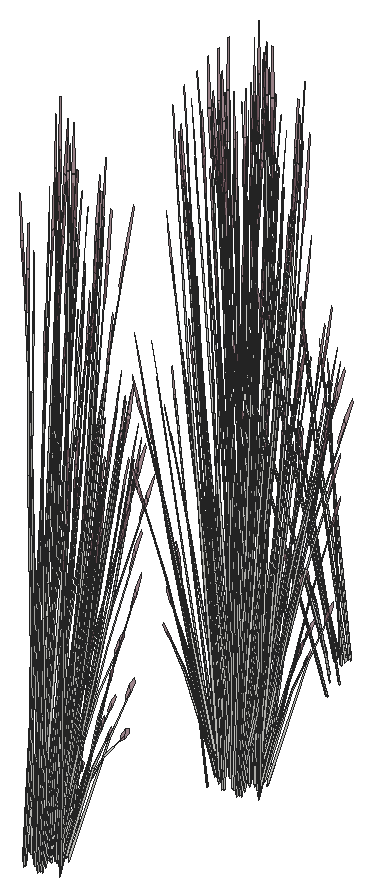
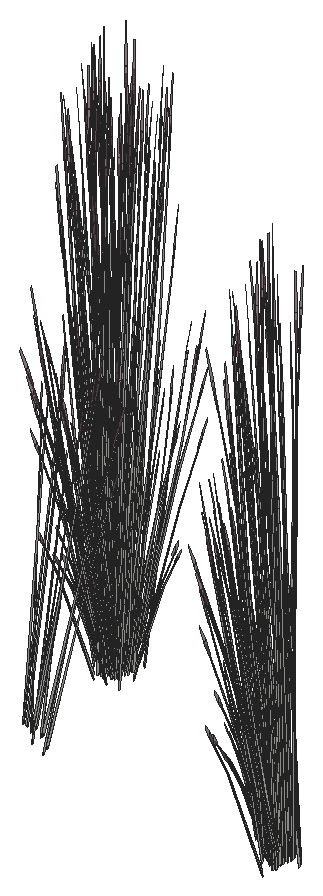
# SketchUp Ruby script. Lengths in inches.
U = 1.inch
M = Sketchup.active_model
def pt(a) = Geom::Point3d.new(a.map { |v| v * U })
def face(e, loops, mat)
  f = e.add_face(loops[0].map { |a| pt(a) })
  loops[1..].each { |l| e.add_face(l.map { |a| pt(a) }).erase! }
  f.material = f.back_material = mat if mat
  f
end
# faces: each face lists its corners as indices into pts; further lists are holes
def faces(e, pts, list, mat = nil) = list.each { |f| face(e, (f[0].is_a?(Array) ? f : [f]).map { |l| l.map { |i| pts[i] } }, mat) }
# xy, xz, yz: faces in a plane at the given z, y or x. An outline is a flat list of corners, or four numbers for a rectangle; further outlines are holes
def ring(l) = l.size == 4 ? [[l[0], l[1]], [l[2], l[1]], [l[2], l[3]], [l[0], l[3]]] : l.each_slice(2).to_a
def flat(e, list, mat, &to3) = list.each { |f| face(e, (f[0].is_a?(Array) ? f : [f]).map { |l| ring(l).map { |u, v| to3.(u, v) } }, mat) }
def xy(e, z, list, mat = nil) = flat(e, list, mat) { |x, y| [x, y, z] }
def xz(e, y, list, mat = nil) = flat(e, list, mat) { |x, z| [x, y, z] }
def yz(e, x, list, mat = nil) = flat(e, list, mat) { |y, z| [x, y, z] }
def lines(e, pts, list) = list.each { |a, b| e.add_line(pt(pts[a]), pt(pts[b])) }
# prism: a flat outline (further loops are holes) pulled along v
def prism(e, loops, v, mat = nil)
  f = face(e, loops, mat); d = Geom::Vector3d.new(v.map { |x| x * U })
  f.pushpull(f.normal.samedirection?(d) ? d.length : -d.length)
end
def box(e, o, s, mat = nil) = prism(e, [[o, [o[0] + s[0], o[1], o[2]], [o[0] + s[0], o[1] + s[1], o[2]], [o[0], o[1] + s[1], o[2]]]], [0, 0, s[2]], mat)
def at(x, y, z, deg = 0) = Geom::Transformation.translation(pt([x, y, z])) * Geom::Transformation.rotation(ORIGIN, Z_AXIS, deg.degrees)
def axes(o, x, y, z) = Geom::Transformation.new([*x, 0, *y, 0, *z, 0, *pt(o).to_a, 1])
def part(name) = M.definitions.add(name)
# library, detail: a bought-in or finely detailed component or shape, given as its bounding box
def library(name, o, s) = part(name).tap { |d| box(d.entities, o, s) }
def detail(e, o, s) = box(e.add_group.entities, o, s)
def put(e, d, t, mat = nil) = e.add_instance(d, t).tap { |i| i.material = mat if mat }
def group(e, t, mat = nil) = e.add_group.tap { |g| g.transformation = t; g.material = mat if mat }.entities
root = M.entities
M.materials.add("LightPink_Translucent").color = [144, 107, 117]
M.materials["LightPink_Translucent"].alpha = 0.75
c1 = part("blade")
p = [[2.15,0.21,22],[0,0.17,0],[0.09,0.45,0],[2.18,0.31,22],[2.29,0.31,22],[0.38,0.45,0],
  [2.48,0.24,33],[2.49,0.24,33],[2.48,0.22,33]]
faces(c1.entities,p,[[0,1,2,3],[4,5,2,3],[6,3,4,7],[8,0,3,6]])
c2 = part("seeds")
p = [[0.3,-0.1,1.38],[-0.01,-0.03,1.59],[-0.01,-0.03,0.03],[0.14,-0.07,-0.07],[0.29,-0.03,3],[0.15,0.01,3.11]]
faces(c2.entities,p,[[0,1,2,3],[1,0,4,5]],"LightPink_Translucent")
c3 = part("blade with seeds")
put(c3.entities,c1,at(0,0,0))
put(c3.entities,c2,axes([2.4,0.25,30.99],[1.5799,-0.05474,1.17369],[-0.12525,1.92788,0.29478],[-0.07173,-0.02425,1.56792]))
put(root,c3,axes([400.68,21.1,4.53],[-0.20082,-0.29199,-0.35414],[0.2293,-0.2764,0.4572],[-0.1165,-0.04206,0.87481]))
put(root,c3,axes([382.84,21.97,-10.55],[-0.04113,-0.53214,-0.29095],[0.42835,-0.03218,-0.50002],[0.07543,-0.07088,1.59708]))
put(root,c3,axes([401.86,21.97,2.67],[-0.04113,-0.53214,-0.29095],[0.42835,-0.03218,-0.50002],[0.07543,-0.07088,1.59708]))
put(root,c3,axes([400.8,22,2.03],[0.24637,-0.29097,-0.30978],[0.24637,0.29097,0.30978],[0,-0.09372,1.38974]))
put(root,c3,axes([400.7,20.6,2.13],[-0.10181,0.3808,-0.03893],[-0.31336,-0.11714,-0.17649],[-0.04758,-0.06228,0.58215]))
put(root,c3,axes([384.39,21.85,-8.16],[-0.30722,0.06665,0.35414],[-0.08112,-0.381,-0.4572],[0.08804,-0.10234,0.87481]))
put(root,c3,axes([401.67,22.53,2.67],[-0.39748,-0.22252,-0.29095],[0.19139,-0.46966,-0.50002],[-0.01249,-0.11531,1.59708]))
put(root,c3,axes([400.53,22.34,2.375],[-0.44133,0,0],[0,-0.52122,-0.51607],[0,-0.11871,1.63711]))
put(root,c3,axes([400.61,21.41,2.59],[0.06891,0.12984,1.43002],[-0.15879,0.35293,-0.30754],[-0.16304,-0.08436,0.61141]))
put(root,c3,axes([382.78,20.79,-11.18],[0.32928,0.11539,-0.30978],[-0.08291,0.40636,0.30978],[0.06638,-0.04686,1.38974]))
put(root,c3,axes([401.81,20.79,2.03],[0.32928,0.11539,-0.30978],[-0.08291,0.40636,0.30978],[0.06638,-0.04686,1.38974]))
put(root,c3,axes([400.89,21.29,4.98],[-0.35281,-0.01123,-0.71045],[0.0237,-0.47284,0.08574],[-0.14947,-0.0499,1.00501]))
put(root,c3,axes([384.67,21.79,-8.48],[0.2423,0.19613,0.0643],[-0.14107,0.2793,0.50621],[0.07768,-0.0903,0.77189]))
put(root,c3,axes([384.6,21.71,-8.48],[0.08753,0.42921,0.48003],[-0.34336,0.07449,0.3958],[0.1012,-0.10094,0.9933]))
put(root,c3,axes([385.53,22.22,-8.5],[0.04898,-0.07104,1.74944],[-0.06269,-0.43574,-0.27667],[0.12289,-0.08262,0.14031]))
put(root,c3,axes([400.875,22.2,2.33],[-0.32829,0.39208,0.30756],[-0.32849,-0.38796,-0.36492],[-0.01146,-0.11134,1.64885]))
put(root,c3,axes([382.89,22.39,-10.78],[0.39767,0.22603,0.24065],[-0.19139,0.46966,0.50002],[0,-0.10827,1.60543]))
put(root,c3,axes([401.92,22.39,2.43],[0.39767,0.22603,0.24065],[-0.19139,0.46966,0.50002],[0,-0.10827,1.60543]))
put(root,c3,axes([401.77,23.02,2.4375],[0.09355,-0.55261,-0.23429],[0.44354,0.09633,0.51271],[-0.0775,-0.07631,1.5644]))
put(root,c3,axes([400.78,21.39,4.68],[-0.25628,0.30892,-0.51099],[-0.22444,-0.32634,-0.3958],[-0.13021,-0.047,0.97773]))
put(root,c3,axes([400.2,21.8,2.77],[0.22533,-0.03337,1.1486],[-0.14293,0.29403,0.84392],[-0.11135,-0.04411,0.25299]))
put(root,c3,axes([382.76,22.07,-10.49],[-0.38326,0.02879,0.44739],[-0.03466,-0.47788,-0.21531],[0.06861,-0.04843,1.43643]))
put(root,c3,axes([401.79,22.07,2.72],[-0.38326,0.02879,0.44739],[-0.03466,-0.47788,-0.21531],[0.06861,-0.04843,1.43643]))
put(root,c3,axes([400.8,22.42,2.48],[0,0.46636,0.49651],[-0.39487,0,0],[0,-0.10622,1.57504]))
put(root,c3,axes([384.5625,22.89,-8.18],[-0.17758,-0.42229,-0.1216],[0.31518,-0.20752,-0.67495],[0.13282,-0.05572,1.02557]))
put(root,c3,axes([384.55,22.52,-8.53],[0.09562,-0.42421,-0.51099],[0.32782,0.1454,-0.3958],[0.13199,-0.0389,0.97773]))
put(root,c3,axes([403.57,22.52,4.68],[0.09562,-0.42421,-0.51099],[0.32782,0.1454,-0.3958],[0.13199,-0.0389,0.97773]))
put(root,c3,axes([384.03,20.8,-10.83],[0.22066,-0.46731,0],[0.36918,0.26061,-0.51607],[0.08408,0.05936,1.63711]))
put(root,c3,axes([403.06,20.8,2.375],[0.22066,-0.46731,0],[0.36918,0.26061,-0.51607],[0.08408,0.05936,1.63711]))
put(root,c3,axes([400.46,21.72,3.875],[0.14639,-0.01056,1.71376],[-0.09712,0.45778,0.13857],[-0.20862,-0.02831,0.73262]))
put(root,c3,axes([401.73,22.8,2.21],[-0.21202,-0.39143,-0.44739],[0.32115,-0.27564,0.21531],[-0.06861,-0.04843,1.43643]))
put(root,c3,axes([401.78,22.24,2.36],[0.15345,0.52148,0.45755],[-0.43845,0.18134,0.17955],[0.00536,-0.09582,1.58856]))
put(root,c3,axes([384.9,22.64,-11.23],[-0.22732,0.05597,1.41583],[-0.03618,-0.44548,0.08104],[0.15921,-0.06743,0.80566]))
put(root,c3,axes([403.92,22.64,1.98],[-0.22732,0.05597,1.41583],[-0.03618,-0.44548,0.08104],[0.15921,-0.06743,0.80566]))
put(root,c3,axes([385.31,22.25,-10.95],[-0.21881,-0.29821,-0.06488],[0.23965,-0.27324,-0.29416],[0.0679,-0.01924,0.97024]))
put(root,c3,axes([404.34,22.25,2.26],[-0.21881,-0.29821,-0.06488],[0.23965,-0.27324,-0.29416],[0.0679,-0.01924,0.97024]))
put(root,c3,axes([401.7,22.65,2.72],[-0.17124,0.42022,0.44739],[-0.35581,-0.20224,-0.21531],[0,-0.09687,1.43643]))
put(root,c3,axes([402.33,22.29,2.21],[0,-0.53961,0],[0.44133,0,0],[0,0,1.79456]))
put(root,c3,axes([383.84,21.04,-10.73],[-0.33032,-0.23318,0.49651],[0.19744,-0.41812,0],[0.07523,0.05311,1.57504]))
put(root,c3,axes([402.87,21.04,2.48],[-0.33032,-0.23318,0.49651],[0.19744,-0.41812,0],[0.07523,0.05311,1.57504]))
put(root,c3,axes([384.48,22.68,-8.23],[0.31014,-0.20596,-0.71045],[0.17284,0.42397,0.08574],[0.14985,-0.04816,1.00501]))
put(root,c3,axes([403.51,22.68,4.98],[0.31014,-0.20596,-0.71045],[0.17284,0.42397,0.08574],[0.14985,-0.04816,1.00501]))
put(root,c3,axes([401.54,22.95,2.06],[-0.36714,-0.07646,-0.62353],[0.07747,-0.47163,-0.16365],[-0.10956,-0.05715,1.37633]))
put(root,c3,axes([383.09,21.95,-10.85],[-0.29264,0.42323,0.45755],[-0.34767,-0.3736,0.17955],[0.07055,-0.04224,1.58856]))
put(root,c3,axes([402.12,21.95,2.36],[-0.29264,0.42323,0.45755],[-0.34767,-0.3736,0.17955],[0.07055,-0.04224,1.58856]))
put(root,c3,axes([402.44,22.71,2.3],[-0.32829,-0.4014,-0.06131],[0.32849,-0.40164,0],[-0.01146,-0.01402,1.75571]))
put(root,c3,axes([382.58,21.25,-10.74],[-0.10196,0.46348,0.17642],[-0.3731,-0.13116,0.35086],[0.06445,-0.00226,1.60407]))
put(root,c3,axes([401.61,21.25,2.47],[-0.10196,0.46348,0.17642],[-0.3731,-0.13116,0.35086],[0.06445,-0.00226,1.60407]))
put(root,c3,axes([384.4375,22.76,-8.16],[-0.29332,-0.1301,0.35414],[0.08555,-0.37955,-0.4572],[0.11809,-0.0348,0.87481]))
put(root,c3,axes([382.43,21.625,-11.62],[-0.3474,0.18671,1.28929],[-0.11057,-0.53572,0.50096],[0.21332,0.00891,1.46642]))
put(root,c3,axes([401.46,21.625,1.59],[-0.3474,0.18671,1.28929],[-0.11057,-0.53572,0.50096],[0.21332,0.00891,1.46642]))
put(root,c3,axes([383.36,21.77,-10.59],[0.06809,-0.4162,0.1448],[0.33266,0.07225,-0.41347],[0.06054,0.04274,1.26744]))
put(root,c3,axes([402.39,21.77,2.62],[0.06809,-0.4162,0.1448],[0.33266,0.07225,-0.41347],[0.06054,0.04274,1.26744]))
put(root,c3,axes([401.82,22.75,2.36],[0.44609,0.09826,0.45755],[-0.09078,0.55493,0.17955],[-0.06519,-0.05359,1.58856]))
put(root,c3,axes([385.14,22.35,-11.72],[-0.01845,-0.0708,1.76342],[0.12793,-0.41416,-0.26939],[0.12905,-0.00596,0.30037]))
put(root,c3,axes([404.17,22.35,1.49],[-0.01845,-0.0708,1.76342],[0.12793,-0.41416,-0.26939],[0.12905,-0.00596,0.30037]))
put(root,c3,axes([400.36,22.28,1.49],[0.00895,0.0735,1.76342],[-0.18044,0.38382,-0.26939],[-0.12817,-0.01935,0.30037]))
put(root,c3,axes([383.22,21.875,-10.49],[-0.21202,-0.39143,0.44739],[0.32115,-0.27564,-0.21531],[0.06861,0.04843,1.43643]))
put(root,c3,axes([402.25,21.875,2.72],[-0.21202,-0.39143,0.44739],[0.32115,-0.27564,-0.21531],[0.06861,0.04843,1.43643]))
put(root,c3,axes([401.15,23.66,2.03],[-0.08291,-0.40636,-0.30978],[0.32928,-0.11539,0.30978],[-0.06638,-0.04686,1.38974]))
put(root,c3,axes([401.58,23.64,2.47],[0.37926,-0.12378,0.17642],[0.09365,0.46065,0.35086],[-0.03382,-0.06712,1.60407]))
put(root,c3,axes([383.33,21.9,-10.55],[0.35635,-0.30962,-0.29095],[0.23697,0.43749,-0.50002],[0.08792,0.04443,1.59708]))
put(root,c3,axes([402.36,21.9,2.67],[0.35635,-0.30962,-0.29095],[0.23697,0.43749,-0.50002],[0.08792,0.04443,1.59708]))
put(root,c3,axes([384.75,22.72,-8.68],[0.29332,0.1301,-0.35414],[-0.08555,0.37955,0.4572],[0.11809,-0.0348,0.87481]))
put(root,c3,axes([403.78,22.72,4.53],[0.29332,0.1301,-0.35414],[-0.08555,0.37955,0.4572],[0.11809,-0.0348,0.87481]))
put(root,c3,axes([401.0625,23.84,2.02],[-0.33032,-0.23318,-0.49651],[0.19744,-0.41812,0],[-0.07523,-0.05311,1.57504]))
put(root,c3,axes([384.23,21.08,-11.19],[0.33032,0.23318,-0.49651],[-0.19744,0.41812,0],[0.07523,0.05311,1.57504]))
put(root,c3,axes([403.26,21.08,2.02],[0.33032,0.23318,-0.49651],[-0.19744,0.41812,0],[0.07523,0.05311,1.57504]))
put(root,c3,axes([400.33,22.11,4.53],[-0.29332,-0.1301,-0.35414],[0.08555,-0.37955,0.4572],[-0.11809,0.0348,0.87481]))
put(root,c3,axes([383.6,22.41,-11.01],[0.39487,0,0],[0,0.48281,0],[0,0,1.78407]))
put(root,c3,axes([402.63,22.41,2.21],[0.39487,0,0],[0,0.48281,0],[0,0,1.78407]))
put(root,c3,axes([401.96,23.02,2.67],[-0.35635,0.30962,-0.29095],[-0.23697,-0.43749,-0.50002],[-0.08792,-0.04443,1.59708]))
put(root,c3,axes([383.71,21.28,-10.74],[-0.37926,0.12378,0.17642],[-0.09365,-0.46065,0.35086],[0.03382,0.06712,1.60407]))
put(root,c3,axes([402.74,21.28,2.47],[-0.37926,0.12378,0.17642],[-0.09365,-0.46065,0.35086],[0.03382,0.06712,1.60407]))
put(root,c3,axes([383.95,22.25,-9.33],[-0.14639,0.01056,1.71376],[0.09712,-0.45778,0.13857],[0.20862,0.02831,0.73262]))
put(root,c3,axes([402.98,22.25,3.875],[-0.14639,0.01056,1.71376],[0.09712,-0.45778,0.13857],[0.20862,0.02831,0.73262]))
put(root,c3,axes([384.14,21.25,-11.18],[0.08291,0.40636,-0.30978],[-0.32928,0.11539,0.30978],[0.06638,0.04686,1.38974]))
put(root,c3,axes([403.17,21.25,2.03],[0.08291,0.40636,-0.30978],[-0.32928,0.11539,0.30978],[0.06638,0.04686,1.38974]))
put(root,c3,axes([384.7,22.875,-8.48],[0.12963,0.31798,0.0643],[-0.23638,0.15564,0.50621],[0.1042,-0.03071,0.77189]))
put(root,c3,axes([383.47,22.16,-10.83],[-0.44609,-0.09826,0.49198],[0.09078,-0.55493,0.19306],[0.06519,0.05359,1.70813]))
put(root,c3,axes([402.5,22.16,2.38],[-0.44609,-0.09826,0.49198],[0.09078,-0.55493,0.19306],[0.06519,0.05359,1.70813]))
put(root,c3,axes([384.68,22.76,-8.48],[-0.09971,0.42522,0.48003],[-0.32782,-0.1454,0.3958],[0.12892,-0.02555,0.9933]))
put(root,c3,axes([402.15,23.53,2.2],[-0.11516,-0.40207,0],[0.32884,-0.1408,0],[0,0,1.54371]))
put(root,c3,axes([401.93,23.15,2.62],[-0.06809,0.4162,0.1448],[-0.33266,-0.07225,-0.41347],[-0.06054,-0.04274,1.26744]))
put(root,c3,axes([383.55,23.48,-11.03],[0.37054,-0.15823,-0.19198],[0.1302,0.45581,0.00008],[0.0409,-0.01749,1.73897]))
put(root,c3,axes([402.58,23.48,2.18],[0.37054,-0.15823,-0.19198],[0.1302,0.45581,0.00008],[0.0409,-0.01749,1.73897]))
put(root,c3,axes([402.71,23.67,2.47],[0.10196,-0.46348,0.17642],[0.3731,0.13116,0.35086],[-0.06445,0.00226,1.60407]))
put(root,c3,axes([383.59,22.62,-11],[0.24637,0.30123,0],[-0.24637,0.30123,0],[0,0,1.69266]))
put(root,c3,axes([402.62,22.62,2.21],[0.24637,0.30123,0],[-0.24637,0.30123,0],[0,0,1.69266]))
put(root,c3,axes([401.22,22.05,3.34],[0.10032,-0.06746,1.77064],[0.0346,0.47103,0.13857],[-0.2173,0.0625,0.63284]))
put(root,c3,axes([403.29,22.48,2.47],[-0.2773,-0.3397,0.17642],[0.27945,-0.32949,0.35086],[-0.03063,0.06937,1.60407]))
put(root,c3,axes([383.75,21.97,-11.15],[0.36714,0.07646,-0.62353],[-0.07747,0.47163,-0.16365],[0.10956,0.05715,1.37633]))
put(root,c3,axes([402.78,21.97,2.06],[0.36714,0.07646,-0.62353],[-0.07747,0.47163,-0.16365],[0.10956,0.05715,1.37633]))
put(root,c3,axes([385.37,22.79,-10.45],[-0.21807,0.07699,1.1486],[0.10265,-0.31819,0.84392],[0.11568,0.02177,0.25299]))
put(root,c3,axes([404.4,22.79,2.77],[-0.21807,0.07699,1.1486],[0.10265,-0.31819,0.84392],[0.11568,0.02177,0.25299]))
put(root,c3,axes([402.07,23.71,2.2],[-0.35581,-0.20937,0],[0.17124,-0.43505,0],[0,0,1.62707]))
put(root,c3,axes([402.36,23.16,2.46],[-0.34464,-0.37536,-0.25192],[0.29,-0.42149,0.5513],[-0.0928,0.04391,1.68216]))
put(root,c3,axes([401.45,23.875,2.48],[0.33032,0.23318,0.49651],[-0.19744,0.41812,0],[-0.07523,-0.05311,1.57504]))
put(root,c3,axes([383.59,22.26,-10.49],[0.17124,-0.42022,0.44739],[0.35581,0.20224,-0.21531],[0,0.09687,1.43643]))
put(root,c3,axes([402.62,22.26,2.72],[0.17124,-0.42022,0.44739],[0.35581,0.20224,-0.21531],[0,0.09687,1.43643]))
put(root,c3,axes([385.27,24.14,-8.5],[-0.03191,-0.04083,1.77383],[0.06981,-0.43764,-0.16761],[0.12571,-0.02796,0.31391]))
put(root,c3,axes([383.52,22.5,-10.92],[0,0.53934,-0.05637],[-0.44133,0,0],[0,0.01695,1.79368]))
put(root,c3,axes([402.55,22.5,2.29],[0,0.53934,-0.05637],[-0.44133,0,0],[0,0.01695,1.79368]))
put(root,c3,axes([400.53,22.31,4.68],[-0.09562,0.42421,-0.51099],[-0.32782,-0.1454,-0.3958],[-0.13199,0.0389,0.97773]))
put(root,c3,axes([383.56,22.12,-11],[0.21202,0.39143,-0.44739],[-0.32115,0.27564,0.21531],[0.06861,0.04843,1.43643]))
put(root,c3,axes([402.58,22.12,2.21],[0.21202,0.39143,-0.44739],[-0.32115,0.27564,0.21531],[0.06861,0.04843,1.43643]))
put(root,c3,axes([384.99,23.78,-9.28],[-0.06755,-0.39203,-0.03492],[0.31928,-0.09013,-0.15832],[0.06667,0.02485,0.52218]))
put(root,c3,axes([404.02,23.78,3.93],[-0.06755,-0.39203,-0.03492],[0.31928,-0.09013,-0.15832],[0.06667,0.02485,0.52218]))
put(root,c3,axes([401.26,24.12,2.375],[-0.22066,0.46731,0],[-0.36918,-0.26061,-0.51607],[-0.08408,-0.05936,1.63711]))
put(root,c3,axes([384.16,23.76,-8.18],[0.0189,-0.47427,-0.1216],[0.35781,0.01296,-0.67495],[0.13781,0.03295,1.02557]))
put(root,c3,axes([384.49,22.5,-10.73],[0,-0.46636,0.49651],[0.39487,0,0],[0,0.10622,1.57504]))
put(root,c3,axes([403.52,22.5,2.48],[0,-0.46636,0.49651],[0.39487,0,0],[0,0.10622,1.57504]))
put(root,c3,axes([402.53,22.85,2.72],[0.38326,-0.02879,0.44739],[0.03466,0.47788,-0.21531],[-0.06861,0.04843,1.43643]))
put(root,c3,axes([383.74,22.36,-10.59],[0.32884,-0.136,0.1448],[0.11516,0.38837,-0.41347],[0,0.08547,1.26744]))
put(root,c3,axes([402.77,22.36,2.62],[0.32884,-0.136,0.1448],[0.11516,0.38837,-0.41347],[0,0.08547,1.26744]))
put(root,c3,axes([384.11,23.58,-8.16],[-0.20082,-0.29199,0.35414],[0.2293,-0.2764,-0.4572],[0.1165,0.04206,0.87481]))
put(root,c3,axes([402.1875,23.08,2.21],[-0.38326,0.02879,-0.44739],[-0.03466,-0.47788,0.21531],[-0.06861,0.04843,1.43643]))
put(root,c3,axes([384.96,23.3,-10.62],[-0.085,-0.1147,1.43002],[0.1106,-0.37943,-0.30754],[0.17198,0.0514,0.61141]))
put(root,c3,axes([403.99,23.3,2.59],[-0.085,-0.1147,1.43002],[0.1106,-0.37943,-0.30754],[0.17198,0.0514,0.61141]))
put(root,c3,axes([383.44,23.72,-11.01],[0.35581,0.20937,0],[-0.17124,0.43505,0],[0,0,1.74954]))
put(root,c3,axes([402.47,23.72,2.2],[0.35581,0.20937,0],[-0.17124,0.43505,0],[0,0,1.74954]))
put(root,c3,axes([384.47,23.48,-8.5],[0.07571,-0.00789,1.74944],[0.20767,-0.36231,-0.27667],[0.13467,0.04783,0.14031]))
put(root,c3,axes([402.61,24.19,2.19],[-0.21791,-0.46895,-0.05142],[0.36918,-0.26061,0.51607],[-0.09097,0.04465,1.6363]))
put(root,c3,axes([402.53,23.05,2.62],[0.26075,0.2802,0.1448],[-0.2175,0.31612,-0.41347],[-0.06054,0.04274,1.26744]))
put(root,c3,axes([400.52,22.52,3.875],[0.12246,-0.09864,1.71376],[0.1031,0.45582,0.13857],[-0.19225,0.10302,0.73262]))
put(root,c3,axes([384.18,23.54,-8.23],[0.35281,0.01123,-0.71045],[-0.0237,0.47284,0.08574],[0.14947,0.0499,1.00501]))
put(root,c3,axes([403.21,23.54,4.98],[0.35281,0.01123,-0.71045],[-0.0237,0.47284,0.08574],[0.14947,0.0499,1.00501]))
put(root,c3,axes([402.8125,23.91,2.48],[0.33032,-0.23318,0.49651],[0.19744,0.41812,0],[-0.07523,0.05311,1.57504]))
put(root,c3,axes([383.3125,23.55,-10.92],[0.15345,0.53576,-0.06012],[-0.43845,0.18773,0],[0.00536,0.01871,1.72173]))
put(root,c3,axes([402.34,23.55,2.29],[0.15345,0.53576,-0.06012],[-0.43845,0.18773,0],[0.00536,0.01871,1.72173]))
put(root,c3,axes([402.51,24.125,2.03],[-0.32928,-0.11539,-0.30978],[0.08291,-0.40636,0.30978],[-0.06638,0.04686,1.38974]))
put(root,c3,axes([400.14,23.3,2.59],[0.12266,0.03828,1.43002],[0.07906,0.39104,-0.30754],[-0.16661,0.0732,0.61141]))
put(root,c3,axes([384.76,22.58,-10.83],[0.44133,0,0],[0,0.52122,-0.51607],[0,0.11871,1.63711]))
put(root,c3,axes([403.78,22.58,2.375],[0.44133,0,0],[0,0.52122,-0.51607],[0,0.11871,1.63711]))
put(root,c3,axes([384.58,22.84,-11.01],[-0.44111,-0.00373,-0.04976],[0,-0.52122,0.49943],[-0.01386,0.11865,1.58352]))
put(root,c3,axes([403.61,22.84,2.2],[-0.44111,-0.00373,-0.04976],[0,-0.52122,0.49943],[-0.01386,0.11865,1.58352]))
put(root,c3,axes([383.625,22.39,-10.55],[0.39748,0.22252,-0.29095],[-0.19139,0.46966,-0.50002],[0.01249,0.11531,1.59708]))
put(root,c3,axes([402.65,22.39,2.67],[0.39748,0.22252,-0.29095],[-0.19139,0.46966,-0.50002],[0.01249,0.11531,1.59708]))
put(root,c3,axes([399.88,24.12,2.77],[0.14709,-0.21136,1.1486],[0.05804,0.3346,0.84392],[-0.1063,0.05991,0.25299]))
put(root,c3,axes([384.39,23.73,-8.68],[0.20082,0.29199,-0.35414],[-0.2293,0.2764,0.4572],[0.1165,0.04206,0.87481]))
put(root,c3,axes([403.42,23.73,4.53],[0.20082,0.29199,-0.35414],[-0.2293,0.2764,0.4572],[0.1165,0.04206,0.87481]))
put(root,c3,axes([384.49,22.92,-11.18],[-0.24637,0.29097,-0.30978],[-0.24637,-0.29097,0.30978],[0,0.09372,1.38974]))
put(root,c3,axes([403.52,22.92,2.03],[-0.24637,0.29097,-0.30978],[-0.24637,-0.29097,0.30978],[0,0.09372,1.38974]))
put(root,c3,axes([402.46,22.95,2.67],[0.04113,0.53214,-0.29095],[-0.42835,0.03218,-0.50002],[-0.07543,0.07088,1.59708]))
put(root,c3,axes([384.29,23.84,-8.48],[-0.01777,0.35463,0.0643],[-0.26836,-0.00972,0.50621],[0.1028,0.03711,0.77189]))
put(root,c3,axes([402.61,22.74,2.21],[-0.17124,0.42022,-0.44739],[-0.35581,-0.20224,0.21531],[0,0.09687,1.43643]))
put(root,c3,axes([400.43,23.21,4.53],[-0.30722,0.06665,-0.35414],[-0.08112,-0.381,0.4572],[-0.08804,0.10234,0.87481]))
put(root,c3,axes([384.3125,23.73,-8.48],[-0.26024,0.30729,0.48003],[-0.22444,-0.32634,0.3958],[0.1221,0.05668,0.9933]))
put(root,c3,axes([402.2,23.35,2.06],[-0.23773,0.35053,-0.62353],[-0.29532,-0.31785,-0.16365],[-0.09526,0.08744,1.37633]))
put(root,c3,axes([383.49,24.09,-8.16],[-0.05451,-0.37564,0.35414],[0.31161,-0.09919,-0.4572],[0.0837,0.10765,0.87481]))
put(root,c3,axes([402.62,23.94,2.33],[0.44186,0.15158,0.30756],[-0.11054,0.54181,-0.36492],[-0.07313,0.06781,1.64885]))
put(root,c3,axes([402.59,24.31,2.02],[-0.33032,0.23318,-0.49651],[-0.19744,-0.41812,0],[-0.07523,0.05311,1.57504]))
put(root,c3,axes([384.66,22.93,-11.19],[0,0.46636,-0.49651],[-0.39487,0,0],[0,0.10622,1.57504]))
put(root,c3,axes([403.6875,22.93,2.02],[0,0.46636,-0.49651],[-0.39487,0,0],[0,0.10622,1.57504]))
put(root,c3,axes([383.67,22.98,-9.33],[-0.1311,-0.08035,1.71376],[0.27131,-0.33708,0.13857],[0.16909,0.15206,0.73262]))
put(root,c3,axes([402.7,22.98,3.875],[-0.1311,-0.08035,1.71376],[0.27131,-0.33708,0.13857],[0.16909,0.15206,0.73262]))
put(root,c3,axes([383.7,21.92,-8.74],[-0.30498,-0.24231,1.38283],[0.32203,-0.37727,0.59665],[0.0984,0.22736,1.33663]))
put(root,c3,axes([384.16,23.9,-10.45],[-0.19872,-0.13409,1.1486],[0.2566,-0.13625,0.84392],[0.06921,0.11541,0.25299]))
put(root,c3,axes([403.18,23.9,2.77],[-0.19872,-0.13409,1.1486],[0.2566,-0.13625,0.84392],[0.06921,0.11541,0.25299]))
put(root,c3,axes([383.46,24.28,-8.18],[0.21031,-0.39918,-0.1216],[0.30457,0.22997,-0.67495],[0.10587,0.11278,1.02557]))
put(root,c3,axes([400.97,22.83,3.875],[0.08815,-0.14329,1.71376],[0.22258,0.38678,0.13857],[-0.15267,0.17614,0.73262]))
put(root,c3,axes([400.6875,23.25,4.68],[0.09067,0.42583,-0.51099],[-0.34336,0.07449,-0.3958],[-0.0984,0.11438,0.97773]))
put(root,c3,axes([402.89,24.24,2.375],[0.22066,0.46731,0],[-0.36918,0.26061,-0.51607],[-0.08408,0.05936,1.63711]))
put(root,c3,axes([383.18,24.61,-8.5],[0.00104,-0.05646,1.77383],[0.30246,-0.2491,-0.16761],[0.10506,0.08891,0.31391]))
put(root,c3,axes([384.21,24.4,-11.72],[0.02571,-0.06733,1.76342],[0.32373,-0.19829,-0.26939],[0.09815,0.10263,0.30037]))
put(root,c3,axes([403.24,24.4,1.49],[0.02571,-0.06733,1.76342],[0.32373,-0.19829,-0.26939],[0.09815,0.10263,0.30037]))
put(root,c3,axes([402.7,22.39,2.84],[-0.00964,-0.43909,1.41272],[0.43635,0.11382,0.59816],[-0.1032,0.24027,1.3335]))
put(root,c3,axes([383.78,22.87,-11.12],[0.12941,0.42699,-0.69212],[-0.37279,0.15378,-0.18165],[0.0143,0.14459,1.52773]))
put(root,c3,axes([402.8125,22.87,2.09],[0.12941,0.42699,-0.69212],[-0.37279,0.15378,-0.18165],[0.0143,0.14459,1.52773]))
put(root,c3,axes([400.27,24.34,1.49],[0.04734,0.04659,1.76342],[0.08027,0.4317,-0.26939],[-0.10492,0.09206,0.30037]))
put(root,c3,axes([383.71,24.08,-8.53],[0.34827,-0.11086,-0.51099],[0.06092,0.41983,-0.3958],[0.09354,0.12031,0.97773]))
put(root,c3,axes([402.74,24.08,4.68],[0.34827,-0.11086,-0.51099],[0.06092,0.41983,-0.3958],[0.09354,0.12031,0.97773]))
put(root,c3,axes([382.74,24.14,-8.16],[0.1064,-0.35863,0.35414],[0.31043,0.1046,-0.4572],[0.02846,0.14439,0.87481]))
put(root,c3,axes([384.1875,24.51,-10.54],[-0.22633,-0.01463,1.0506],[0.14947,-0.31064,0.58006],[0.08941,0.11036,0.8241]))
put(root,c3,axes([403.22,24.51,2.67],[-0.22633,-0.01463,1.0506],[0.14947,-0.31064,0.58006],[0.08941,0.11036,0.8241]))
put(root,c3,axes([383.54,24.43,-8.48],[-0.16041,0.29625,0.0643],[-0.22843,-0.17248,0.50621],[0.07385,0.09498,0.77189]))
put(root,c3,axes([383.16,25.42,-7.56],[0.2439,-0.26754,-0.06488],[0.22348,0.29302,-0.29416],[0.01573,0.08303,0.97024]))
put(root,c3,axes([383.6,24.34,-8.48],[-0.35104,0.10702,0.48003],[-0.06092,-0.41983,0.3958],[0.08256,0.12373,0.9933]))
put(root,c3,axes([400.9,23.19,3.875],[0.06572,-0.16029,1.71376],[0.27569,0.33172,0.13857],[-0.12437,0.20675,0.73262]))
put(root,c3,axes([383.45,23.75,-10.62],[0.00623,-0.15459,1.43002],[0.29764,-0.17268,-0.30754],[0.09188,0.18503,0.61141]))
put(root,c3,axes([402.48,23.75,2.59],[0.00623,-0.15459,1.43002],[0.29764,-0.17268,-0.30754],[0.09188,0.18503,0.61141]))
put(root,c3,axes([400.98,24.09,4.53],[-0.23881,0.24554,-0.35414],[-0.22606,-0.28036,0.4572],[-0.0344,0.14245,0.87481]))
put(root,c3,axes([382.64,24.3,-8.18],[0.34538,-0.21713,-0.1216],[0.16972,0.38536,-0.67495],[0.04557,0.16239,1.02557]))
put(root,c3,axes([401.13,25.04,2.77],[-0.00913,-0.2773,1.1486],[0.22824,0.19778,0.84392],[-0.04489,0.13217,0.25299]))
put(root,c3,axes([401.73,24.38,1.49],[0.05712,-0.02538,1.76342],[0.34359,0.13968,-0.26939],[0.01005,0.15742,0.30037]))
put(root,c3,axes([401.21,23.97,5],[0.25266,0.31335,-0.5672],[-0.2669,0.27442,-0.43934],[-0.03844,0.15921,1.08528]))
put(root,c3,axes([400.9375,24.44,2.82],[0.32063,-0.08258,0.06507],[0.07371,0.33271,-0.86304],[-0.02033,0.16842,0.7736]))
put(root,c3,axes([382.93,24.28,-8.53],[0.34695,0.11691,-0.51099],[-0.11892,0.40083,-0.3958],[0.03181,0.16138,0.97773]))
put(root,c3,axes([401.96,24.28,4.68],[0.34695,0.11691,-0.51099],[-0.11892,0.40083,-0.3958],[0.03181,0.16138,0.97773]))
put(root,c3,axes([383.13,23.45,-9.33],[-0.08068,-0.14973,1.71376],[0.3728,-0.12606,0.13857],[0.08426,0.23506,0.73262]))
put(root,c3,axes([402.16,23.45,3.875],[-0.08068,-0.14973,1.71376],[0.3728,-0.12606,0.13857],[0.08426,0.23506,0.73262]))
put(root,c3,axes([401.8,24.52,4.53],[-0.1064,0.35863,-0.35414],[-0.31043,-0.1046,0.4572],[0.02846,0.14439,0.87481]))
put(root,c3,axes([401.13,23.83,5.34],[-0.00918,0.43138,-0.7886],[-0.38672,-0.02897,0.09517],[-0.04081,0.18275,1.11556]))
put(root,c3,axes([401.5,23.52,3.875],[-0.00864,-0.17899,1.71376],[0.37441,0.11874,0.13857],[-0.02316,0.25508,0.73262]))
put(root,c3,axes([382.81,24.2,-8.23],[0.16845,0.3792,-0.71045],[-0.34676,0.21133,0.08574],[0.03939,0.18322,1.00501]))
put(root,c3,axes([401.84,24.2,4.98],[0.16845,0.3792,-0.71045],[-0.34676,0.21133,0.08574],[0.03939,0.18322,1.00501]))
put(root,c3,axes([400.86,24.8,2.59],[0.11138,-0.07357,1.43002],[0.27499,0.22183,-0.30754],[-0.08185,0.19194,0.61141]))
put(root,c3,axes([401.01,24.4375,3.36],[0.00775,-0.24075,1.54345],[0.34877,0.12716,0.21329],[-0.03022,0.25658,0.72882]))
put(root,c3,axes([397.68,38.5625,3.875],[0.08068,0.14973,1.71376],[-0.3728,0.12606,0.13857],[-0.08426,-0.23506,0.73262]))
put(root,c3,axes([399.13,38.35,2.59],[-0.10032,0.0944,1.43002],[-0.30046,-0.16522,-0.30754],[0.05569,-0.20547,0.61141]))
put(root,c3,axes([398.67,38.68,4.98],[-0.16845,-0.3792,-0.71045],[0.34676,-0.21133,0.08574],[-0.03939,-0.18322,1.00501]))
put(root,c3,axes([397.57,38.17,2.59],[-0.02137,0.15256,1.43002],[-0.31245,0.12771,-0.30754],[-0.07303,-0.19719,0.61141]))
put(root,c3,axes([398.38,37.83,1.49],[-0.0592,0.0168,1.76342],[-0.32738,-0.18913,-0.26939],[0.00549,-0.15776,0.30037]))
put(root,c3,axes([399.37,39.05,4.98],[0.00918,-0.43138,-0.71045],[0.38672,0.02897,0.08574],[0.04081,-0.18275,1.00501]))
put(root,c3,axes([398.7,38.35,4.53],[0.1064,-0.35863,-0.35414],[0.31043,0.1046,0.4572],[-0.02846,-0.14439,0.87481]))
put(root,c3,axes([398.9375,38.83,3.875],[-0.06572,0.16029,1.71376],[-0.27569,-0.33172,0.13857],[0.12437,-0.20675,0.73262]))
put(root,c3,axes([398.54,38.6,4.68],[-0.34695,-0.11691,-0.51099],[0.11892,-0.40083,-0.3958],[-0.03181,-0.16138,0.97773]))
put(root,c3,axes([398.76,37.6,2.77],[0.04528,0.27194,1.1486],[-0.25117,-0.15062,0.84392],[0.02703,-0.13924,0.25299]))
put(root,c3,axes([399.29,38.9,4.68],[-0.25266,-0.31335,-0.51099],[0.2669,-0.27442,-0.3958],[0.03844,-0.15921,0.97773]))
put(root,c3,axes([399.53,38.79,4.53],[0.23881,-0.24554,-0.35414],[0.22606,0.28036,0.4572],[0.0344,-0.14245,0.87481]))
